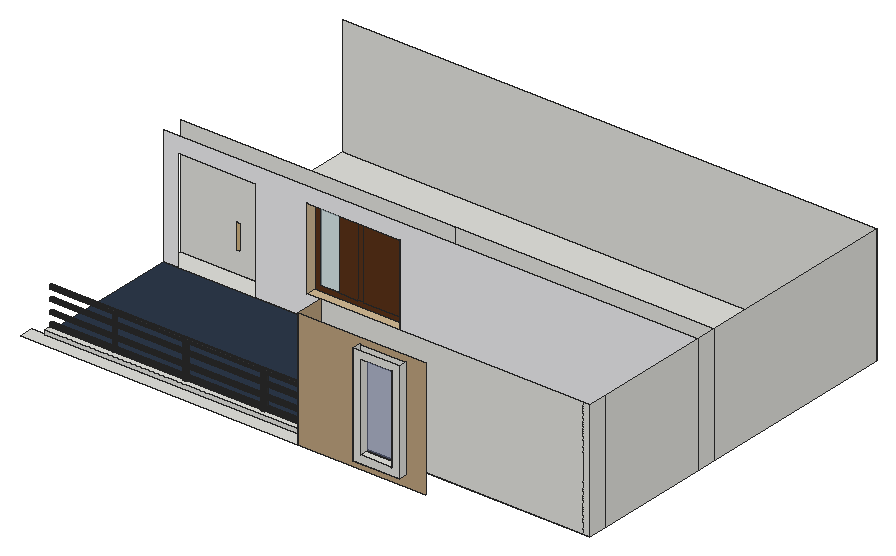
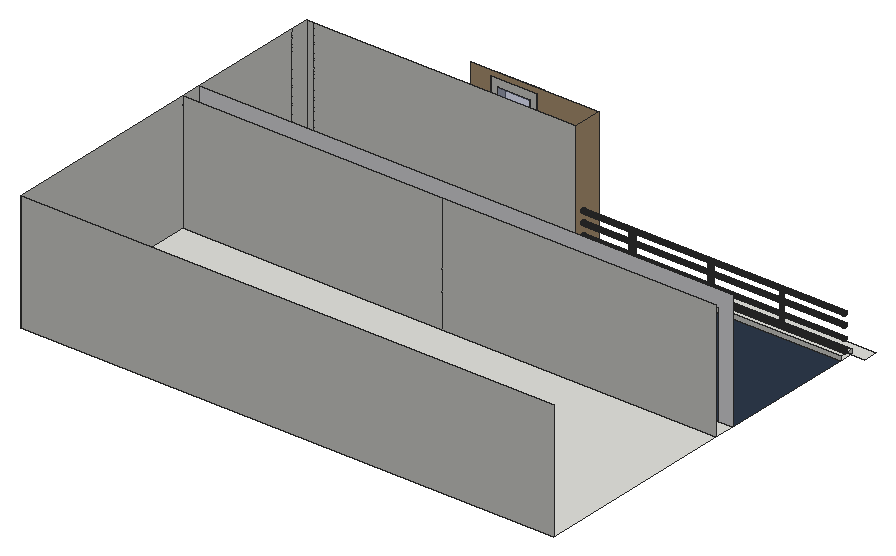
# SketchUp Ruby script. Lengths in inches.
U = 1.inch
M = Sketchup.active_model
def pt(a) = Geom::Point3d.new(a.map { |v| v * U })
def face(e, loops, mat)
  f = e.add_face(loops[0].map { |a| pt(a) })
  loops[1..].each { |l| e.add_face(l.map { |a| pt(a) }).erase! }
  f.material = f.back_material = mat if mat
  f
end
# faces: each face lists its corners as indices into pts; further lists are holes
def faces(e, pts, list, mat = nil) = list.each { |f| face(e, (f[0].is_a?(Array) ? f : [f]).map { |l| l.map { |i| pts[i] } }, mat) }
# xy, xz, yz: faces in a plane at the given z, y or x. An outline is a flat list of corners, or four numbers for a rectangle; further outlines are holes
def ring(l) = l.size == 4 ? [[l[0], l[1]], [l[2], l[1]], [l[2], l[3]], [l[0], l[3]]] : l.each_slice(2).to_a
def flat(e, list, mat, &to3) = list.each { |f| face(e, (f[0].is_a?(Array) ? f : [f]).map { |l| ring(l).map { |u, v| to3.(u, v) } }, mat) }
def xy(e, z, list, mat = nil) = flat(e, list, mat) { |x, y| [x, y, z] }
def xz(e, y, list, mat = nil) = flat(e, list, mat) { |x, z| [x, y, z] }
def yz(e, x, list, mat = nil) = flat(e, list, mat) { |y, z| [x, y, z] }
def lines(e, pts, list) = list.each { |a, b| e.add_line(pt(pts[a]), pt(pts[b])) }
# prism: a flat outline (further loops are holes) pulled along v
def prism(e, loops, v, mat = nil)
  f = face(e, loops, mat); d = Geom::Vector3d.new(v.map { |x| x * U })
  f.pushpull(f.normal.samedirection?(d) ? d.length : -d.length)
end
def box(e, o, s, mat = nil) = prism(e, [[o, [o[0] + s[0], o[1], o[2]], [o[0] + s[0], o[1] + s[1], o[2]], [o[0], o[1] + s[1], o[2]]]], [0, 0, s[2]], mat)
def at(x, y, z, deg = 0) = Geom::Transformation.translation(pt([x, y, z])) * Geom::Transformation.rotation(ORIGIN, Z_AXIS, deg.degrees)
def axes(o, x, y, z) = Geom::Transformation.new([*x, 0, *y, 0, *z, 0, *pt(o).to_a, 1])
def part(name) = M.definitions.add(name)
# library, detail: a bought-in or finely detailed component or shape, given as its bounding box
def library(name, o, s) = part(name).tap { |d| box(d.entities, o, s) }
def detail(e, o, s) = box(e.add_group.entities, o, s)
def put(e, d, t, mat = nil) = e.add_instance(d, t).tap { |i| i.material = mat if mat }
def group(e, t, mat = nil) = e.add_group.tap { |g| g.transformation = t; g.material = mat if mat }.entities
root = M.entities
M.materials.add("[0035_Tan]").color = [188, 161, 125]
M.materials.add("[Blinds Vertical Pattern]").color = [237, 237, 239]
M.materials.add("[Color M07]").color = [58, 58, 58]
M.materials.add("[Formica Beige]").color = [211, 187, 149]
M.materials.add("[Leather Blue]").color = [45, 57, 74]
M.materials.add("[Translucent Glass Safety]").color = [204, 235, 244]
M.materials["[Translucent Glass Safety]"].alpha = 0.5
M.materials.add("[Translucent Glass Sky Reflection]").color = [126, 138, 183]
M.materials["[Translucent Glass Sky Reflection]"].alpha = 0.52
M.materials.add("[Wood Cherry Original]").color = [89, 50, 24]
M.materials.add("[Wood Floor Light]").color = [204, 176, 127]
xy(root,276.4375,[[73.92,393.34,320.99,405.6875],[[85.98,405.6875,320.99,418.04],[206.33,409.67,206.96,409.75,207.55,409.97,208.0625,410.32,208.45,410.77,208.7,411.3,208.78,411.86,208.7,412.43,208.45,412.96,208.0625,413.41,207.55,413.76,206.96,413.98,206.33,414.05,205.69,413.98,205.1,413.76,204.6,413.41,204.21,412.96,203.96,412.43,203.88,411.86,203.96,411.3,204.21,410.77,204.6,410.32,205.1,409.97,205.69,409.75],[275.91,409.67,276.54,409.75,277.13,409.97,277.64,410.32,278.03,410.77,278.28,411.3,278.36,411.86,278.28,412.43,278.03,412.96,277.64,413.41,277.13,413.76,276.54,413.98,275.91,414.05,275.27,413.98,274.68,413.76,274.18,413.41,273.79,412.96,273.54,412.43,273.46,411.86,273.54,411.3,273.79,410.77,274.18,410.32,274.68,409.97,275.27,409.75],[142,409.67,142.63,409.75,143.22,409.97,143.73,410.32,144.12,410.77,144.37,411.3,144.45,411.86,144.37,412.43,144.12,412.96,143.73,413.41,143.22,413.76,142.63,413.98,142,414.05,141.36,413.98,140.77,413.76,140.27,413.41,139.875,412.96,139.63,412.43,139.55,411.86,139.63,411.3,139.875,410.77,140.27,410.32,140.77,409.97,141.36,409.75]],[206.33,409.67,205.69,409.75,205.1,409.97,204.6,410.32,204.21,410.77,203.96,411.3,203.88,411.86,203.96,412.43,204.21,412.96,204.6,413.41,205.1,413.76,205.69,413.98,206.33,414.05,206.96,413.98,207.55,413.76,208.0625,413.41,208.45,412.96,208.7,412.43,208.78,411.86,208.7,411.3,208.45,410.77,208.0625,410.32,207.55,409.97,206.96,409.75],[275.91,409.67,275.27,409.75,274.68,409.97,274.18,410.32,273.79,410.77,273.54,411.3,273.46,411.86,273.54,412.43,273.79,412.96,274.18,413.41,274.68,413.76,275.27,413.98,275.91,414.05,276.54,413.98,277.13,413.76,277.64,413.41,278.03,412.96,278.28,412.43,278.36,411.86,278.28,411.3,278.03,410.77,277.64,410.32,277.13,409.97,276.54,409.75],[85.98,538.2,560.26,556.28],
  [85.98,556.28,560.26,737.09]])
xy(root,276.4375,[[85.98,418.04,560.26,538.2]],"[Leather Blue]")
xy(root,280.5,[[[85.98,405.6875,320.99,418.04],[206.33,409.67,205.69,409.75,205.1,409.97,204.6,410.32,204.21,410.77,203.96,411.3,203.88,411.86,203.96,412.43,204.21,412.96,204.6,413.41,205.1,413.76,205.69,413.98,206.33,414.05,206.96,413.98,207.55,413.76,208.0625,413.41,208.45,412.96,208.7,412.43,208.78,411.86,208.7,411.3,208.45,410.77,208.0625,410.32,207.55,409.97,206.96,409.75],[275.91,409.67,275.27,409.75,274.68,409.97,274.18,410.32,273.79,410.77,273.54,411.3,273.46,411.86,273.54,412.43,273.79,412.96,274.18,413.41,274.68,413.76,275.27,413.98,275.91,414.05,276.54,413.98,277.13,413.76,277.64,413.41,278.03,412.96,278.28,412.43,278.36,411.86,278.28,411.3,278.03,410.77,277.64,410.32,277.13,409.97,276.54,409.75],[142,409.67,141.36,409.75,140.77,409.97,140.27,410.32,139.875,410.77,139.63,411.3,139.55,411.86,139.63,412.43,139.875,412.96,140.27,413.41,140.77,413.76,141.36,413.98,142,414.05,142.63,413.98,143.22,413.76,143.73,413.41,144.12,412.96,144.37,412.43,144.45,411.86,144.37,411.3,144.12,410.77,143.73,410.32,143.22,409.97,142.63,409.75]]])
xy(root,286.61,[[375.85,385.97,417.04,393.34]])
xy(root,293.02,[[382.27,385.97,410.625,393.34]])
xy(root,295.11,[[212.94,538.2,295.68,547.45]],"[Formica Beige]")
xy(root,311.375,[[206.33,409.67,206.96,409.75,207.55,409.97,208.0625,410.32,208.45,410.77,208.7,411.3,208.78,411.86,208.7,412.43,208.45,412.96,208.0625,413.41,207.55,413.76,206.96,413.98,206.33,414.05,205.69,413.98,205.1,413.76,204.6,413.41,204.21,412.96,203.96,412.43,203.88,411.86,203.96,411.3,204.21,410.77,204.6,410.32,205.1,409.97,205.69,409.75]])
xy(root,311.5,[[275.91,409.67,276.54,409.75,277.13,409.97,277.64,410.32,278.03,410.77,278.28,411.3,278.36,411.86,278.28,412.43,278.03,412.96,277.64,413.41,277.13,413.76,276.54,413.98,275.91,414.05,275.27,413.98,274.68,413.76,274.18,413.41,273.79,412.96,273.54,412.43,273.46,411.86,273.54,411.3,273.79,410.77,274.18,410.32,274.68,409.97,275.27,409.75]])
xz(root,385.97,[[[375.85,286.61,417.04,376.36],[382.27,293.02,410.625,369.94]]])
xz(root,393.34,[[[375.85,286.61,417.04,376.36],[382.27,293.02,410.625,369.94]]])
xz(root,393.34,[[[320.99,276.4375,434.25,381.625],[375.85,286.61,417.04,376.36]]],"[0035_Tan]")
xz(root,393.34,[[382.27,293.02,410.625,369.94]],"[Translucent Glass Sky Reflection]")
xz(root,405.6875,[[85.98,276.4375,320.99,280.5]])
xz(root,418.04,[[85.98,276.4375,320.99,280.5],[320.99,276.4375,554.62,381.625],[554.62,276.4375,560.26,381.625]])
xz(root,538.2,[[[85.98,276.4375,98.05,276.4375,98.05,367.3125,167.49,367.3125,167.49,276.4375,560.26,276.4375,560.26,381.625,85.98,381.625],[212.94,295.11,295.68,367.68]]],"[Blinds Vertical Pattern]")
xz(root,538.2,[[150.45,308.77,153.53,330.52]],"[Wood Floor Light]")
xz(root,547.45,[[217.71,299.38,234.47,363.41]],"[Translucent Glass Safety]")
xz(root,547.45,[[[212.94,295.11,295.68,367.68],[217.71,299.38,290.9,363.41]],[234.47,299.38,251.22,363.41],[251.22,299.38,256.24,363.41],[256.24,299.38,290.9,363.41]],"[Wood Cherry Original]")
xz(root,556.28,[[85.98,276.4375,329.72,381.625],[329.72,276.4375,560.26,381.625]])
xz(root,737.09,[[85.98,276.4375,560.26,381.625]])
yz(root,212.94,[[538.2,295.11,547.45,367.68]],"[Formica Beige]")
yz(root,295.68,[[538.2,295.11,547.45,367.68]],"[Formica Beige]")
yz(root,320.99,[[405.6875,276.4375,405.6875,280.5,411,280.5,411.03,280.46,411.4,280.18,411.82,280.01,412.27,279.95,412.72,280.01,413.15,280.18,413.51,280.46,413.54,280.5,418.04,280.5,418.04,276.4375],[412.27,279.95,412.72,280.01,413.15,280.18,413.51,280.46,413.54,280.5,411,280.5,411.03,280.46,411.4,280.18,411.82,280.01]])
yz(root,320.99,[[[393.34,276.4375,393.34,381.625,418.04,381.625,418.04,280.5,413.54,280.5,413.79,280.82,413.96,281.24,414.02,281.7,413.96,282.15,413.79,282.57,413.51,282.93,413.15,283.21,412.72,283.39,412.27,283.45,411.82,283.39,411.4,283.21,411.03,282.93,410.76,282.57,410.58,282.15,410.52,281.7,410.58,281.24,410.76,280.82,411,280.5,405.6875,280.5,405.6875,276.4375],[412.27,309.95,412.72,310.01,413.15,310.18,413.51,310.46,413.79,310.82,413.96,311.24,414.02,311.7,413.96,312.15,413.79,312.57,413.51,312.93,413.15,313.21,412.72,313.39,412.27,313.45,411.82,313.39,411.4,313.21,411.03,312.93,410.76,312.57,410.58,312.15,410.52,311.7,410.58,311.24,410.76,310.82,411.03,310.46,411.4,310.18,411.82,310.01],[412.27,300.26,412.72,300.32,413.15,300.49,413.51,300.77,413.79,301.13,413.96,301.56,414.02,302.01,413.96,302.46,413.79,302.88,413.51,303.25,413.15,303.53,412.72,303.7,412.27,303.76,411.82,303.7,411.4,303.53,411.03,303.25,410.76,302.88,410.58,302.46,410.52,302.01,410.58,301.56,410.76,301.13,411.03,300.77,411.4,300.49,411.82,300.32],[412.27,289.88,412.72,289.94,413.15,290.12,413.51,290.4,413.79,290.76,413.96,291.18,414.02,291.63,413.96,292.09,413.79,292.51,413.51,292.87,413.15,293.15,412.72,293.33,412.27,293.38,411.82,293.33,411.4,293.15,411.03,292.87,410.76,292.51,410.58,292.09,410.52,291.63,410.58,291.18,410.76,290.76,411.03,290.4,411.4,290.12,411.82,289.94]]],"[0035_Tan]")
yz(root,375.85,[[385.97,286.61,393.34,376.36]])
yz(root,382.27,[[385.97,293.02,393.34,369.94]])
yz(root,410.625,[[385.97,293.02,393.34,369.94]])
yz(root,417.04,[[385.97,286.61,393.34,376.36]])
yz(root,560.26,[[418.04,276.4375,434.85,381.625],[434.85,276.4375,538.2,381.625],[538.2,276.4375,556.28,381.625],[556.28,276.4375,737.09,381.625]])
p = [[205.1,409.97,276.4375],[205.69,409.75,276.4375],[205.69,409.75,280.5],[205.1,409.97,280.5],[206.33,409.67,276.4375],[206.33,409.67,280.5],
  [206.96,409.75,276.4375],[206.96,409.75,280.5],[207.55,409.97,276.4375],[207.55,409.97,280.5],[274.68,409.97,276.4375],[275.27,409.75,276.4375],
  [275.27,409.75,280.5],[274.68,409.97,280.5],[275.91,409.67,276.4375],[275.91,409.67,280.5],[276.54,409.75,276.4375],[276.54,409.75,280.5],
  [277.13,409.97,276.4375],[277.13,409.97,280.5],[204.6,410.32,276.4375],[204.6,410.32,280.5],[208.0625,410.32,276.4375],[208.0625,410.32,280.5],
  [274.18,410.32,276.4375],[274.18,410.32,280.5],[277.64,410.32,276.4375],[277.64,410.32,280.5],[143.73,410.32,276.4375],[144.12,410.77,276.4375],
  [144.12,410.77,280.5],[143.73,410.32,280.5],[204.21,410.77,276.4375],[204.21,410.77,280.5],[208.45,410.77,276.4375],[208.45,410.77,280.5],
  [273.79,410.77,276.4375],[273.79,410.77,280.5],[278.03,410.77,276.4375],[278.03,410.77,280.5],[144.37,411.3,276.4375],[144.37,411.3,280.5],
  [203.96,411.3,276.4375],[203.96,411.3,280.5],[208.7,411.3,276.4375],[208.7,411.3,280.5],[273.54,411.3,276.4375],[273.54,411.3,280.5],
  [278.28,411.3,276.4375],[278.28,411.3,280.5],[144.45,411.86,276.4375],[144.45,411.86,280.5],[203.88,411.86,276.4375],[203.88,411.86,280.5],
  [208.78,411.86,276.4375],[208.78,411.86,280.5],[273.46,411.86,276.4375],[273.46,411.86,280.5],[278.36,411.86,276.4375],[278.36,411.86,280.5],
  [144.37,412.43,276.4375],[144.37,412.43,280.5],[203.96,412.43,276.4375],[203.96,412.43,280.5],[208.7,412.43,276.4375],[208.7,412.43,280.5],
  [273.54,412.43,276.4375],[273.54,412.43,280.5],[278.28,412.43,276.4375],[278.28,412.43,280.5],[144.12,412.96,276.4375],[144.12,412.96,280.5],
  [204.21,412.96,276.4375],[204.21,412.96,280.5],[208.45,412.96,276.4375],[208.45,412.96,280.5],[273.79,412.96,276.4375],[273.79,412.96,280.5],
  [278.03,412.96,276.4375],[278.03,412.96,280.5],[143.73,413.41,276.4375],[143.73,413.41,280.5],[204.6,413.41,276.4375],[204.6,413.41,280.5],
  [208.0625,413.41,276.4375],[208.0625,413.41,280.5],[274.18,413.41,276.4375],[274.18,413.41,280.5],[277.64,413.41,276.4375],[277.64,413.41,280.5],
  [205.1,413.76,276.4375],[205.1,413.76,280.5],[207.55,413.76,276.4375],[207.55,413.76,280.5],[274.68,413.76,276.4375],[274.68,413.76,280.5],
  [277.13,413.76,276.4375],[277.13,413.76,280.5],[205.69,413.98,276.4375],[205.69,413.98,280.5],[206.96,413.98,276.4375],[206.96,413.98,280.5],
  [275.27,413.98,276.4375],[275.27,413.98,280.5],[276.54,413.98,276.4375],[276.54,413.98,280.5],[206.33,414.05,276.4375],[206.33,414.05,280.5],
  [275.91,414.05,276.4375],[275.91,414.05,280.5],[85.98,411.82,280.01],[85.98,412.27,279.95],[320.99,412.27,279.95],[320.99,411.82,280.01],
  [85.98,412.72,280.01],[320.99,412.72,280.01],[85.98,411.4,280.18],[320.99,411.4,280.18],[85.98,413.15,280.18],[320.99,413.15,280.18],
  [85.98,411.03,280.46],[320.99,411.03,280.46],[85.98,413.51,280.46],[320.99,413.51,280.46],[205.1,409.97,311.375],[205.69,409.75,311.375],
  [206.33,409.67,311.375],[206.96,409.75,311.375],[207.55,409.97,311.375],[274.68,409.97,311.5],[275.27,409.75,311.5],[275.91,409.67,311.5],
  [276.54,409.75,311.5],[277.13,409.97,311.5],[143.22,409.97,311.3125],[143.22,409.97,280.5],[143.73,410.32,311.3125],[204.6,410.32,311.375],
  [208.0625,410.32,311.375],[274.18,410.32,311.5],[277.64,410.32,311.5],[144.12,410.77,311.3125],[204.21,410.77,311.375],[208.45,410.77,311.375],
  [273.79,410.77,311.5],[278.03,410.77,311.5],[85.98,411,280.5],[320.99,411,280.5],[320.99,410.76,280.82],[85.98,410.76,280.82],
  [144.37,411.3,311.3125],[203.96,411.3,311.375],[208.7,411.3,311.375],[273.54,411.3,311.5],[278.28,411.3,311.5],[144.45,411.86,311.3125],
  [203.88,411.86,311.375],[208.78,411.86,311.375],[273.46,411.86,311.5],[278.36,411.86,311.5],[144.37,412.43,311.3125],[203.96,412.43,311.375],
  [208.7,412.43,311.375],[273.54,412.43,311.5],[278.28,412.43,311.5],[144.12,412.96,311.3125],[204.21,412.96,311.375],[208.45,412.96,311.375],
  [273.79,412.96,311.5],[278.03,412.96,311.5],[143.73,413.41,311.3125],[204.6,413.41,311.375],[208.0625,413.41,311.375],[274.18,413.41,311.5],
  [277.64,413.41,311.5],[143.22,413.76,280.5],[143.22,413.76,311.3125],[205.1,413.76,311.375],[207.55,413.76,311.375],[274.68,413.76,311.5],
  [277.13,413.76,311.5],[85.98,413.54,280.5],[85.98,413.79,280.82],[320.99,413.79,280.82],[320.99,413.54,280.5],[205.69,413.98,311.375],
  [206.96,413.98,311.375],[275.27,413.98,311.5],[276.54,413.98,311.5],[206.33,414.05,311.375],[275.91,414.05,311.5],[85.98,410.58,281.24],
  [320.99,410.58,281.24],[85.98,413.96,281.24],[320.99,413.96,281.24],[85.98,410.52,281.7],[320.99,410.52,281.7],[85.98,414.02,281.7],
  [320.99,414.02,281.7],[85.98,410.58,282.15],[320.99,410.58,282.15],[85.98,413.96,282.15],[320.99,413.96,282.15],[85.98,410.76,282.57],
  [320.99,410.76,282.57],[85.98,413.79,282.57],[320.99,413.79,282.57],[85.98,411.03,282.93],[320.99,411.03,282.93],[85.98,413.51,282.93],
  [320.99,413.51,282.93],[85.98,411.4,283.21],[320.99,411.4,283.21],[85.98,413.15,283.21],[320.99,413.15,283.21],[85.98,411.82,283.39],
  [320.99,411.82,283.39],[85.98,412.72,283.39],[320.99,412.72,283.39],[85.98,412.27,283.45],[320.99,412.27,283.45],[85.98,411.4,290.12],
  [85.98,411.82,289.94],[320.99,411.82,289.94],[320.99,411.4,290.12],[85.98,412.27,289.88],[320.99,412.27,289.88],[85.98,412.72,289.94],
  [320.99,412.72,289.94],[85.98,413.15,290.12],[320.99,413.15,290.12],[85.98,411.03,290.4],[320.99,411.03,290.4],[85.98,413.51,290.4],
  [320.99,413.51,290.4],[85.98,410.76,290.76],[320.99,410.76,290.76],[85.98,413.79,290.76],[320.99,413.79,290.76],[85.98,410.58,291.18],
  [320.99,410.58,291.18],[85.98,413.96,291.18],[320.99,413.96,291.18],[85.98,410.52,291.63],[320.99,410.52,291.63],[85.98,414.02,291.63],
  [320.99,414.02,291.63],[85.98,410.58,292.09],[320.99,410.58,292.09],[85.98,413.96,292.09],[320.99,413.96,292.09],[85.98,410.76,292.51],
  [320.99,410.76,292.51],[85.98,413.79,292.51],[320.99,413.79,292.51],[85.98,411.03,292.87],[320.99,411.03,292.87],[85.98,413.51,292.87],
  [320.99,413.51,292.87],[85.98,411.4,293.15],[320.99,411.4,293.15],[85.98,413.15,293.15],[320.99,413.15,293.15],[85.98,411.82,293.33],
  [320.99,411.82,293.33],[85.98,412.72,293.33],[320.99,412.72,293.33],[85.98,412.27,293.38],[320.99,412.27,293.38],[85.98,411.4,300.49],
  [85.98,411.82,300.32],[320.99,411.82,300.32],[320.99,411.4,300.49],[85.98,412.27,300.26],[320.99,412.27,300.26],[85.98,412.72,300.32],
  [320.99,412.72,300.32],[85.98,413.15,300.49],[320.99,413.15,300.49],[85.98,411.03,300.77],[320.99,411.03,300.77],[85.98,413.51,300.77],
  [320.99,413.51,300.77],[85.98,410.76,301.13],[320.99,410.76,301.13],[85.98,413.79,301.13],[320.99,413.79,301.13],[85.98,410.58,301.56],
  [320.99,410.58,301.56],[85.98,413.96,301.56],[320.99,413.96,301.56],[85.98,410.52,302.01],[320.99,410.52,302.01],[85.98,414.02,302.01],
  [320.99,414.02,302.01],[85.98,410.58,302.46],[320.99,410.58,302.46],[85.98,413.96,302.46],[320.99,413.96,302.46],[85.98,410.76,302.88],
  [320.99,410.76,302.88],[85.98,413.79,302.88],[320.99,413.79,302.88],[85.98,411.03,303.25],[320.99,411.03,303.25],[85.98,413.51,303.25],
  [320.99,413.51,303.25],[85.98,411.4,303.53],[320.99,411.4,303.53],[85.98,413.15,303.53],[320.99,413.15,303.53],[85.98,411.82,303.7],
  [320.99,411.82,303.7],[85.98,412.72,303.7],[320.99,412.72,303.7],[85.98,412.27,303.76],[320.99,412.27,303.76],[85.98,411.82,310.01],
  [85.98,412.27,309.95],[320.99,412.27,309.95],[320.99,411.82,310.01],[85.98,412.72,310.01],[320.99,412.72,310.01],[85.98,411.4,310.18],
  [320.99,411.4,310.18],[85.98,413.15,310.18],[320.99,413.15,310.18],[85.98,411.03,310.46],[320.99,411.03,310.46],[85.98,413.51,310.46],
  [320.99,413.51,310.46],[85.98,410.76,310.82],[320.99,410.76,310.82],[85.98,413.79,310.82],[320.99,413.79,310.82],[85.98,410.58,311.24],
  [320.99,410.58,311.24],[85.98,413.96,311.24],[320.99,413.96,311.24],[85.98,410.52,311.7],[320.99,410.52,311.7],[85.98,414.02,311.7],
  [320.99,414.02,311.7],[85.98,410.58,312.15],[320.99,410.58,312.15],[85.98,413.96,312.15],[320.99,413.96,312.15],[85.98,410.76,312.57],
  [320.99,410.76,312.57],[85.98,413.79,312.57],[320.99,413.79,312.57],[85.98,411.03,312.93],[320.99,411.03,312.93],[85.98,413.51,312.93],
  [320.99,413.51,312.93],[85.98,411.4,313.21],[320.99,411.4,313.21],[85.98,413.15,313.21],[320.99,413.15,313.21],[85.98,411.82,313.39],
  [320.99,411.82,313.39],[85.98,412.72,313.39],[320.99,412.72,313.39],[85.98,412.27,313.45],[320.99,412.27,313.45]]
faces(root,p,[[0,1,2,3],[1,4,5,2],[4,6,7,5],[6,8,9,7],[10,11,12,13],[11,14,15,12],[14,16,17,15],[16,18,19,17],
  [20,0,3,21],[8,22,23,9],[24,10,13,25],[18,26,27,19],[28,29,30,31],[32,20,21,33],[22,34,35,23],[36,24,25,37],
  [26,38,39,27],[29,40,41,30],[42,32,33,43],[34,44,45,35],[46,36,37,47],[38,48,49,39],[40,50,51,41],[52,42,43,53],
  [44,54,55,45],[56,46,47,57],[48,58,59,49],[50,60,61,51],[62,52,53,63],[54,64,65,55],[66,56,57,67],[58,68,69,59],
  [60,70,71,61],[72,62,63,73],[64,74,75,65],[76,66,67,77],[68,78,79,69],[70,80,81,71],[82,72,73,83],[74,84,85,75],
  [86,76,77,87],[78,88,89,79],[90,82,83,91],[84,92,93,85],[94,86,87,95],[88,96,97,89],[98,90,91,99],[92,100,101,93],
  [102,94,95,103],[96,104,105,97],[106,98,99,107],[100,106,107,101],[108,102,103,109],[104,108,109,105]])
faces(root,p,[[110,111,112,113],[111,114,115,112],[116,110,113,117],[114,118,119,115],[120,116,117,121],[118,122,123,119],[124,3,2,125],[125,2,5,126],
  [126,5,7,127],[127,7,9,128],[129,13,12,130],[130,12,15,131],[131,15,17,132],[132,17,19,133],[134,135,31,136],[137,21,3,124],
  [128,9,23,138],[139,25,13,129],[133,19,27,140],[136,31,30,141],[142,33,21,137],[138,23,35,143],[144,37,25,139],[140,27,39,145],
  [146,120,121,147,148,149],[141,30,41,150],[151,43,33,142],[143,35,45,152],[153,47,37,144],[145,39,49,154],[150,41,51,155],[156,53,43,151],
  [152,45,55,157],[158,57,47,153],[154,49,59,159],[155,51,61,160],[161,63,53,156],[157,55,65,162],[163,67,57,158],[159,59,69,164],
  [160,61,71,165],[166,73,63,161],[162,65,75,167],[168,77,67,163],[164,69,79,169],[165,71,81,170],[171,83,73,166],[167,75,85,172],
  [173,87,77,168],[169,79,89,174],[170,81,175,176],[177,91,83,171],[172,85,93,178],[179,95,87,173],[174,89,97,180],[181,182,183,184,123,122],
  [185,99,91,177],[178,93,101,186],[187,103,95,179],[180,97,105,188],[189,107,99,185],[186,101,107,189],[190,109,103,187],[188,105,109,190],
  [191,149,148,192],[182,193,194,183],[195,191,192,196],[193,197,198,194],[199,195,196,200],[197,201,202,198],[203,199,200,204],[201,205,206,202],
  [207,203,204,208],[205,209,210,206],[211,207,208,212],[209,213,214,210],[215,211,212,216],[213,217,218,214],[219,215,216,220],[217,219,220,218],
  [221,222,223,224],[222,225,226,223],[225,227,228,226],[227,229,230,228],[231,221,224,232],[229,233,234,230],[235,231,232,236],[233,237,238,234],
  [239,235,236,240],[237,241,242,238],[243,239,240,244],[241,245,246,242],[247,243,244,248],[245,249,250,246],[251,247,248,252],[249,253,254,250],
  [255,251,252,256],[253,257,258,254],[259,255,256,260],[257,261,262,258],[263,259,260,264],[261,265,266,262],[267,263,264,268],[265,267,268,266],
  [269,270,271,272],[270,273,274,271],[273,275,276,274],[275,277,278,276],[279,269,272,280],[277,281,282,278],[283,279,280,284],[281,285,286,282],
  [287,283,284,288],[285,289,290,286],[291,287,288,292],[289,293,294,290],[295,291,292,296],[293,297,298,294],[299,295,296,300],[297,301,302,298],
  [303,299,300,304],[301,305,306,302],[307,303,304,308],[305,309,310,306],[311,307,308,312],[309,313,314,310],[315,311,312,316],[313,315,316,314],
  [317,318,319,320],[318,321,322,319],[323,317,320,324],[321,325,326,322],[327,323,324,328],[325,329,330,326],[331,327,328,332],[329,333,334,330],
  [335,331,332,336],[333,337,338,334],[339,335,336,340],[337,341,342,338],[343,339,340,344],[341,345,346,342],[347,343,344,348],[345,349,350,346],
  [351,347,348,352],[349,353,354,350],[355,351,352,356],[353,357,358,354],[359,355,356,360],[357,361,362,358],[363,359,360,364],[361,363,364,362]],"[Color M07]")
